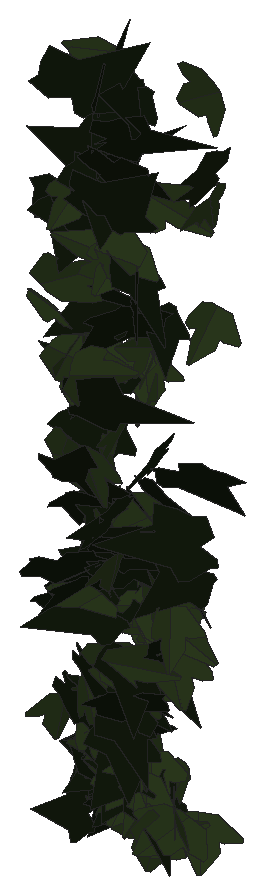
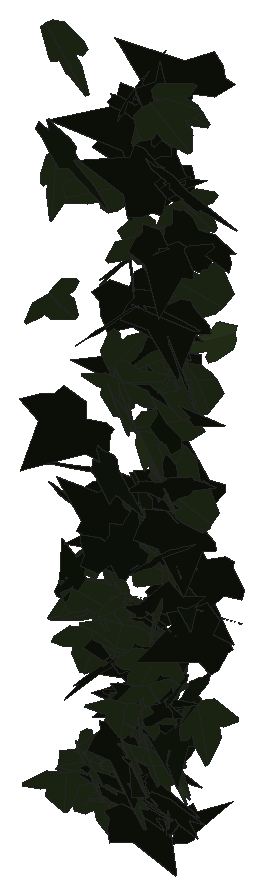
# SketchUp Ruby script. Lengths in inches.
U = 1.inch
M = Sketchup.active_model
def pt(a) = Geom::Point3d.new(a.map { |v| v * U })
def face(e, loops, mat)
  f = e.add_face(loops[0].map { |a| pt(a) })
  loops[1..].each { |l| e.add_face(l.map { |a| pt(a) }).erase! }
  f.material = f.back_material = mat if mat
  f
end
# faces: each face lists its corners as indices into pts; further lists are holes
def faces(e, pts, list, mat = nil) = list.each { |f| face(e, (f[0].is_a?(Array) ? f : [f]).map { |l| l.map { |i| pts[i] } }, mat) }
# xy, xz, yz: faces in a plane at the given z, y or x. An outline is a flat list of corners, or four numbers for a rectangle; further outlines are holes
def ring(l) = l.size == 4 ? [[l[0], l[1]], [l[2], l[1]], [l[2], l[3]], [l[0], l[3]]] : l.each_slice(2).to_a
def flat(e, list, mat, &to3) = list.each { |f| face(e, (f[0].is_a?(Array) ? f : [f]).map { |l| ring(l).map { |u, v| to3.(u, v) } }, mat) }
def xy(e, z, list, mat = nil) = flat(e, list, mat) { |x, y| [x, y, z] }
def xz(e, y, list, mat = nil) = flat(e, list, mat) { |x, z| [x, y, z] }
def yz(e, x, list, mat = nil) = flat(e, list, mat) { |y, z| [x, y, z] }
def lines(e, pts, list) = list.each { |a, b| e.add_line(pt(pts[a]), pt(pts[b])) }
# prism: a flat outline (further loops are holes) pulled along v
def prism(e, loops, v, mat = nil)
  f = face(e, loops, mat); d = Geom::Vector3d.new(v.map { |x| x * U })
  f.pushpull(f.normal.samedirection?(d) ? d.length : -d.length)
end
def box(e, o, s, mat = nil) = prism(e, [[o, [o[0] + s[0], o[1], o[2]], [o[0] + s[0], o[1] + s[1], o[2]], [o[0], o[1] + s[1], o[2]]]], [0, 0, s[2]], mat)
def at(x, y, z, deg = 0) = Geom::Transformation.translation(pt([x, y, z])) * Geom::Transformation.rotation(ORIGIN, Z_AXIS, deg.degrees)
def axes(o, x, y, z) = Geom::Transformation.new([*x, 0, *y, 0, *z, 0, *pt(o).to_a, 1])
def part(name) = M.definitions.add(name)
# library, detail: a bought-in or finely detailed component or shape, given as its bounding box
def library(name, o, s) = part(name).tap { |d| box(d.entities, o, s) }
def detail(e, o, s) = box(e.add_group.entities, o, s)
def put(e, d, t, mat = nil) = e.add_instance(d, t).tap { |i| i.material = mat if mat }
def group(e, t, mat = nil) = e.add_group.tap { |g| g.transformation = t; g.material = mat if mat }.entities
root = M.entities
M.materials.add("1026 AP 7946 SUNNY SIDE UP").color = [254, 231, 186]
M.materials.add("efeu1").color = [18, 25, 13]
M.materials.add("efeu2").color = [43, 57, 29]
c1 = part("ivyleaf_10")
p = [[0,0.5,-0.03],[-0.0625,2.02,-0.43],[-0.19,2.01,-0.46],[-0.54,1.05,-0.29],[-0.52,0.625,-0.18],[-0.83,0.76,-0.28],
  [-1.16,0.64,-0.33],[-1.15,0.33,-0.24],[-0.77,-0.39,0.02],[-0.3,-0.51,0.16],[0.04,-0.48,0.23],[-0.02,2.01,-0.4375],
  [-0.06,2.01,-0.43],[0.04,-0.49,0.23],[0.67,-0.49,0.14],[1.38,0.36,-0.2],[1.375,0.51,-0.24],[0.81,0.65,-0.19],
  [0.62,0.59,-0.15],[0.6,1.09,-0.28],[0.5,1.23,-0.31]]
faces(c1.entities,p,[[0,1,2,3,4,5,6,7,8,9,10],[11,12,0,13,14,15,16,17,18,19,20]],"efeu2")
c2 = part("ivyleaf_9")
p = [[1.54,2.16,1.25],[1.36,2.04,1.19],[-0.21,0.99,0.68],[-0.71,1.11,0.82],[-0.85,0.86,0.67],[-0.8,0.17,0.21],
  [-0.9,-0.01,0.1],[-0.67,-0.16,-0.02],[-0.08,-0.08,-0.05],[-0.03,-0.6,-0.4],[0.65,-0.88,-0.66],[0.83,-0.6,-0.49],
  [1.29,-0.42,-0.43],[1.8125,-0.07,-0.26],[1.21,0.44,0.15]]
faces(c2.entities,p,[[0,1,2,3,4,5,6,7,8,9,10,11,12,13,14]],"efeu1")
put(root,c1,axes([144.89,211.45,272.21],[-0.0227,-0.33557,-0.0993],[-0.00987,0.0948,-0.34531],[0.54808,-0.01219,-0.01033]),"1026 AP 7946 SUNNY SIDE UP")
put(root,c2,axes([144.43,211.41,274.46],[0.30353,0.02891,0.30855],[0.47283,-0.01316,-0.19853],[-0.00717,0.35594,-0.03031]),"1026 AP 7946 SUNNY SIDE UP")
put(root,c2,axes([146.07,211.7,272.7],[-0.47124,0.04372,0.17685],[-0.27106,-0.14791,-0.27249],[0.06248,-0.31197,0.15171]),"1026 AP 7946 SUNNY SIDE UP")
put(root,c1,axes([145.74,211.61,271.51],[0.1198,0.3075,-0.11357],[-0.01937,-0.11221,-0.32669],[-0.51421,0.07587,-0.01416]),"1026 AP 7946 SUNNY SIDE UP")
put(root,c2,axes([144.91,211.76,270.46],[-0.00995,-0.3277,0.08389],[-0.01626,-0.08308,-0.33803],[0.53141,-0.00868,-0.00877]),"1026 AP 7946 SUNNY SIDE UP")
put(root,c2,axes([145.07,211.5,270.11],[0.11535,0.2613,-0.1527],[-0.10067,-0.13703,-0.27952],[-0.4627,0.09496,0.02275]),"1026 AP 7946 SUNNY SIDE UP")
put(root,c2,axes([144.54,211.72,271.16],[-0.46229,-0.00111,0.10729],[-0.1491,-0.12621,-0.27787],[0.06777,-0.28523,0.12054]),"1026 AP 7946 SUNNY SIDE UP")
put(root,c2,axes([144.67,211.55,277.37],[-0.23254,-0.0056,0.30618],[0.43283,-0.12798,0.13786],[0.17658,0.30634,0.0653]),"1026 AP 7946 SUNNY SIDE UP")
put(root,c1,axes([144.78,211.72,276.63],[0.13157,0.14452,0.3287],[-0.29516,-0.25746,0.16978],[0.4636,-0.20493,0.01482]),"1026 AP 7946 SUNNY SIDE UP")
put(root,c1,axes([144.3,211.65,271.27],[0.37111,0.04813,-0.2058],[-0.30199,-0.05766,-0.24807],[-0.11606,0.30396,-0.01258]),"1026 AP 7946 SUNNY SIDE UP")
put(root,c2,axes([144.24,211.68,271.48],[-0.10547,0.19541,-0.2437],[0.01062,-0.24226,-0.20858],[-0.48369,-0.04793,0.04856]),"1026 AP 7946 SUNNY SIDE UP")
put(root,c1,axes([145.05,211.67,268.77],[0.42892,0.15208,-0.10867],[-0.12973,-0.06997,-0.3215],[-0.26138,0.2843,-0.01876]),"1026 AP 7946 SUNNY SIDE UP")
put(root,c1,axes([144.39,211.37,274.9],[-0.06581,-0.08562,-0.35998],[0.30441,0.29057,-0.09567],[0.47593,-0.19769,0.01141]),"1026 AP 7946 SUNNY SIDE UP")
put(root,c2,axes([144.89,211.82,268.94],[-0.30198,-0.20928,0.09031],[-0.03058,-0.10077,-0.28839],[0.3562,-0.18608,0.05181]),"1026 AP 7946 SUNNY SIDE UP")
put(root,c2,axes([143.98,211.61,269.83],[0.32583,-0.23941,-0.09246],[-0.08205,0.07171,-0.32569],[0.39281,0.21357,0.00867]),"1026 AP 7946 SUNNY SIDE UP")
put(root,c1,axes([143.86,211.64,269.62],[-0.14906,-0.31476,-0.00412],[0.02273,-0.00204,-0.33833],[0.49441,-0.0948,0.01431]),"1026 AP 7946 SUNNY SIDE UP")
put(root,c2,axes([144.93,211.82,276.3125],[-0.03483,-0.05751,-0.32695],[0.45525,-0.14301,0.00505],[-0.22234,-0.28381,0.06156]),"1026 AP 7946 SUNNY SIDE UP")
put(root,c2,axes([143.96,211.45,271.84],[0.32103,0.27951,-0.03092],[-0.00381,-0.0373,-0.35621],[-0.44228,0.2032,-0.01937]),"1026 AP 7946 SUNNY SIDE UP")
put(root,c1,axes([144.05,211.74,277.45],[0.23115,0.20832,-0.19197],[-0.16692,-0.1546,-0.26356],[-0.4079,0.18131,-0.00094]),"1026 AP 7946 SUNNY SIDE UP")
put(root,c2,axes([144.76,211.52,272.72],[-0.22638,0.31416,0.00975],[-0.01086,0.00529,-0.35596],[-0.49401,-0.14408,0.00335]),"1026 AP 7946 SUNNY SIDE UP")
put(root,c2,axes([144.18,211.48,279.05],[-0.16959,-0.00997,0.37282],[0.55756,0.07355,0.11137],[-0.11526,0.37045,-0.00982]),"1026 AP 7946 SUNNY SIDE UP")
put(root,c2,axes([144.82,211.78,269.35],[-0.09803,-0.29363,-0.01702],[0.01486,0.01318,-0.30909],[0.46206,-0.06272,0.00633]),"1026 AP 7946 SUNNY SIDE UP")
put(root,c1,axes([144.27,211.64,273.47],[-0.46605,0.12286,-0.0671],[0.07628,-0.0541,-0.32933],[-0.20547,-0.29876,0.02994]),"1026 AP 7946 SUNNY SIDE UP")
put(root,c1,axes([145.75,211.72,268.33],[0.41979,0.05405,-0.17891],[-0.26358,-0.04797,-0.28064],[-0.11216,0.31502,-0.0101]),"1026 AP 7946 SUNNY SIDE UP")
put(root,c1,axes([145.15,211.875,268.51],[-0.09521,-0.19556,0.2531],[0.08334,-0.25406,-0.19548],[0.48806,0.00523,0.08276]),"1026 AP 7946 SUNNY SIDE UP")
put(root,c2,axes([144.98,211.73,275.8125],[-0.04606,0.23487,-0.27374],[-0.03539,-0.26864,-0.24243],[-0.55809,-0.00235,0.03797]),"1026 AP 7946 SUNNY SIDE UP")
put(root,c1,axes([143.45,211.65,275.56],[0.17156,-0.25707,0.06013],[0.39377,0.08037,-0.11424],[0.13112,0.095,0.2644]),"1026 AP 7946 SUNNY SIDE UP")
put(root,c2,axes([146,211.77,272.26],[-0.50513,0.05209,-0.0651],[0.08997,-0.04192,-0.33393],[-0.09263,-0.32477,0.03068]),"1026 AP 7946 SUNNY SIDE UP")
put(root,c2,axes([144.02,211.76,272.95],[0.47426,-0.03134,0.08136],[-0.11757,0.04179,0.31081],[-0.064,-0.30902,0.03193]),"1026 AP 7946 SUNNY SIDE UP")
put(root,c2,axes([144.0625,211.88,267.84],[-0.09074,-0.04802,0.27688],[-0.28488,-0.19915,-0.07782],[0.32173,-0.18988,0.00919]),"1026 AP 7946 SUNNY SIDE UP")
put(root,c1,axes([143.83,211.57,276.02],[-0.20719,-0.15622,0.28667],[0.2926,0.20814,0.2117],[-0.40914,0.22796,0.00623]),"1026 AP 7946 SUNNY SIDE UP")
put(root,c1,axes([144.93,211.48,270.57],[0.12643,0.02144,0.32966],[0.23583,0.28896,-0.0571],[-0.44554,0.15903,0.06333]),"1026 AP 7946 SUNNY SIDE UP")
put(root,c2,axes([144.74,211.8,269.59],[0.05581,-0.29831,-0.02866],[0.0217,0.02791,-0.30883],[0.47036,0.03411,0.01765]),"1026 AP 7946 SUNNY SIDE UP")
put(root,c1,axes([144.3,211.63,269.97],[-0.01626,0.33061,0.03827],[-0.06651,0.0337,-0.33793],[-0.51855,-0.01469,0.04215]),"1026 AP 7946 SUNNY SIDE UP")
put(root,c2,axes([144.12,211.8,268.8],[0.22437,-0.26437,0.01526],[-0.00302,-0.01956,-0.3094],[0.41648,0.14228,-0.01047]),"1026 AP 7946 SUNNY SIDE UP")
put(root,c1,axes([144.63,211.79,269.04],[-0.33322,-0.1935,0.13462],[-0.11605,-0.11345,-0.29458],[0.34934,-0.22226,0.03054]),"1026 AP 7946 SUNNY SIDE UP")
put(root,c1,axes([144.37,211.69,269.4],[0.12774,0.31799,0.00764],[0.02219,0.00218,-0.33782],[-0.49959,0.0814,-0.01305]),"1026 AP 7946 SUNNY SIDE UP")
put(root,c1,axes([144.75,211.84,276.69],[0.29609,0.20892,-0.18212],[-0.16955,-0.14216,-0.29029],[-0.39684,0.21662,-0.01186]),"1026 AP 7946 SUNNY SIDE UP")
put(root,c2,axes([144.93,211.88,268.86],[-0.36004,-0.186,-0.01276],[0.03148,-0.0067,-0.30339],[0.29131,-0.22916,0.01701]),"1026 AP 7946 SUNNY SIDE UP")
put(root,c2,axes([144.98,211.54,272.49],[0.35809,0.25794,0.00745],[0.00483,0.00498,-0.35445],[-0.40566,0.22775,0.00236]),"1026 AP 7946 SUNNY SIDE UP")
put(root,c2,axes([144.36,211.92,277.65],[-0.14218,-0.31337,0.01146],[0.00785,-0.01487,-0.33596],[0.49309,-0.09012,0.00865]),"1026 AP 7946 SUNNY SIDE UP")
put(root,c2,axes([144.33,211.59,271.79],[0.02555,0.31294,0.0444],[-0.06607,0.04315,-0.31939],[-0.49191,0.01046,0.0452]),"1026 AP 7946 SUNNY SIDE UP")
put(root,c2,axes([144.72,211.68,278.07],[0.47008,0.0842,-0.16184],[-0.22483,-0.07141,-0.31919],[-0.16843,0.33031,-0.0256]),"1026 AP 7946 SUNNY SIDE UP")
put(root,c2,axes([144.11,211.77,270.22],[0.35858,-0.2191,-0.0963],[-0.11718,0.05548,-0.32526],[0.35495,0.23965,-0.01009]),"1026 AP 7946 SUNNY SIDE UP")
put(root,c1,axes([145.79,211.67,268.52],[-0.26324,0.22159,0.17373],[-0.2213,0.10078,-0.28188],[-0.37642,-0.21421,0.04422]),"1026 AP 7946 SUNNY SIDE UP")
put(root,c1,axes([145.39,211.625,268.03],[-0.11476,-0.0981,0.29304],[0.18706,0.26006,0.12512],[-0.43547,0.13757,-0.02347]),"1026 AP 7946 SUNNY SIDE UP")
put(root,c2,axes([144.82,211.92,276.47],[0.15948,-0.33075,-0.01898],[-0.02377,0.01266,-0.35615],[0.52018,0.10198,-0.01045]),"1026 AP 7946 SUNNY SIDE UP")
put(root,c2,axes([145.07,211.97,268.34],[0.08236,-0.31394,0.04622],[0.00462,-0.04679,-0.32812],[0.49903,0.05225,-0.00459]),"1026 AP 7946 SUNNY SIDE UP")
put(root,c2,axes([144.83,212.04,278.83],[-0.11578,0.00468,0.32394],[-0.19857,-0.29618,-0.02766],[0.45282,-0.12868,0.07069]),"1026 AP 7946 SUNNY SIDE UP")
put(root,c2,axes([143.7,211.9,277.25],[-0.19955,-0.1001,-0.29884],[0.43708,0.09405,-0.15848],[0.2024,-0.30179,0.0476]),"1026 AP 7946 SUNNY SIDE UP")
put(root,c2,axes([143.87,211.99,276.92],[-0.27109,-0.2359,-0.0123],[0.02941,-0.00056,-0.30059],[0.37014,-0.17273,0.01488]),"1026 AP 7946 SUNNY SIDE UP")
put(root,c1,axes([143.78,211.77,274.84],[-0.19256,-0.06791,-0.29227],[0.44068,0.05652,-0.13843],[0.12518,-0.30344,0.0377]),"1026 AP 7946 SUNNY SIDE UP")
put(root,c2,axes([144.72,211.98,268.86],[-0.43954,-0.0734,0.06198],[-0.08317,-0.03645,-0.29713],[0.12441,-0.28369,0.02034]),"1026 AP 7946 SUNNY SIDE UP")
put(root,c1,axes([145.31,211.86,267.97],[-0.42018,-0.14686,0.06338],[-0.06565,-0.05304,-0.31331],[0.24213,-0.26923,0.02504]),"1026 AP 7946 SUNNY SIDE UP")
put(root,c2,axes([144.44,211.96,275.74],[-0.47524,-0.01458,0.02859],[-0.04087,-0.03536,-0.30996],[0.02777,-0.30145,0.03318]),"1026 AP 7946 SUNNY SIDE UP")
put(root,c1,axes([144.98,211.84,268.9375],[-0.20625,0.26545,-0.02318],[-0.00332,-0.02779,-0.30484],[-0.41908,-0.13042,0.01382]),"1026 AP 7946 SUNNY SIDE UP")
put(root,c2,axes([144.83,211.92,271.72],[0.26227,0.09112,0.25889],[-0.40756,-0.0149,0.18308],[0.09963,-0.30082,0.06742]),"1026 AP 7946 SUNNY SIDE UP")
put(root,c1,axes([144.54,211.92,268.92],[0.44165,0.09446,-0.01587],[-0.00919,-0.0324,-0.30402],[-0.15035,0.27945,-0.02804]),"1026 AP 7946 SUNNY SIDE UP")
put(root,c2,axes([144.83,211.84,270.39],[0.33564,0.22543,0.03474],[-0.06236,-0.00699,0.31885],[0.35265,-0.2158,0.02332]),"1026 AP 7946 SUNNY SIDE UP")
put(root,c1,axes([145.17,211.91,268.96],[0.20195,0.28357,-0.06245],[-0.00767,-0.06593,-0.32026],[-0.45643,0.12657,-0.02225]),"1026 AP 7946 SUNNY SIDE UP")
put(root,c2,axes([144.56,211.69,272.21],[0.08232,0.06124,-0.3348],[0.1751,0.30693,0.07978],[0.49021,-0.11992,0.02773]),"1026 AP 7946 SUNNY SIDE UP")
put(root,c1,axes([144.09,211.91,275.03],[-0.09221,0.29202,-0.06205],[0.00687,-0.06223,-0.3071],[-0.46932,-0.05828,0.0077]),"1026 AP 7946 SUNNY SIDE UP")
put(root,c1,axes([143.76,211.9375,274.59],[-0.04606,-0.31007,0.00879],[0.01913,0.00918,0.3207],[-0.48744,0.02966,0.01176]),"1026 AP 7946 SUNNY SIDE UP")
put(root,c2,axes([144.46,211.73,269.42],[0.02539,0.32457,0.05012],[-0.07478,0.04869,-0.33061],[-0.51019,0.00902,0.05095]),"1026 AP 7946 SUNNY SIDE UP")
put(root,c2,axes([144.6,211.75,278.39],[0.31071,0.03967,0.30087],[0.44369,0.07515,-0.20692],[-0.13262,0.34433,0.01263]),"1026 AP 7946 SUNNY SIDE UP")
put(root,c2,axes([144.02,211.92,274.05],[0.11652,0.25885,0.14764],[-0.09576,-0.12969,0.27584],[0.45414,-0.09376,0.02028]),"1026 AP 7946 SUNNY SIDE UP")
put(root,c1,axes([144.17,212.12,279.17],[-0.1529,-0.13432,0.26367],[-0.16273,-0.23681,-0.16942],[0.4255,-0.13883,0.02995]),"1026 AP 7946 SUNNY SIDE UP")
put(root,c1,axes([143.95,212.1,268.92],[0.20431,-0.22978,0.16112],[0.10531,-0.14316,-0.27257],[0.42538,0.14581,-0.00991]),"1026 AP 7946 SUNNY SIDE UP")
put(root,c1,axes([144.5,212.04,273.79],[0.062,-0.29019,0.05488],[0.00081,-0.05534,-0.30194],[0.46439,0.03884,-0.0068]),"1026 AP 7946 SUNNY SIDE UP")
put(root,c2,axes([144.21,211.9,275.88],[0.32307,0.13237,-0.19886],[-0.25092,-0.11005,-0.25239],[-0.27057,0.26011,-0.00339]),"1026 AP 7946 SUNNY SIDE UP")
put(root,c2,axes([144.91,212.05,269.67],[-0.23811,-0.16435,-0.16914],[-0.19235,-0.10889,0.2292],[-0.30932,0.19423,-0.01232]),"1026 AP 7946 SUNNY SIDE UP")
put(root,c1,axes([144.28,211.85,268.51],[-0.1739,0.17838,0.19408],[-0.22141,0.12945,-0.21181],[-0.34126,-0.17489,0.03852]),"1026 AP 7946 SUNNY SIDE UP")
put(root,c1,axes([144.56,211.88,269.27],[0.17735,0.2207,0.16635],[0.12773,0.13833,-0.25439],[-0.40937,0.13877,-0.0073]),"1026 AP 7946 SUNNY SIDE UP")
put(root,c1,axes([144.73,212,268.86],[-0.42648,0.10548,0.05362],[-0.11532,-0.05118,-0.29047],[-0.14406,-0.27128,0.07376]),"1026 AP 7946 SUNNY SIDE UP")
put(root,c2,axes([144.55,212.14,278.95],[-0.45222,-0.09368,-0.09777],[0.15184,0.00745,-0.31075],[0.14375,-0.30259,0.02067]),"1026 AP 7946 SUNNY SIDE UP")
put(root,c1,axes([144.4,211.99,270.38],[-0.37831,-0.12046,-0.1001],[0.15224,0.02135,-0.27607],[0.18899,-0.25834,0.02201]),"1026 AP 7946 SUNNY SIDE UP")
put(root,c1,axes([144.56,212.03,267.79],[-0.45491,-0.02423,0.08048],[0.11801,0.03678,0.29777],[-0.05165,0.29744,-0.02848]),"1026 AP 7946 SUNNY SIDE UP")
put(root,c1,axes([144.25,212.03,272.17],[-0.40866,0.18256,0.03955],[-0.14741,-0.0727,-0.30637],[-0.25322,-0.2523,0.11452]),"1026 AP 7946 SUNNY SIDE UP")
put(root,c1,axes([143.54,212.05,273.01],[-0.18459,0.00857,0.30537],[0.46592,0.01457,0.12057],[-0.01635,0.31844,-0.01187]),"1026 AP 7946 SUNNY SIDE UP")
put(root,c2,axes([145.71,211.88,273.61],[0.47454,0.15109,0.03882],[0.06461,0.00006,-0.34719],[-0.23584,0.30403,-0.017]),"1026 AP 7946 SUNNY SIDE UP")
put(root,c2,axes([144.5,212.25,268.68],[-0.03475,-0.06692,0.27557],[0.04252,-0.26796,-0.06824],[0.43206,0.02099,0.02888]),"1026 AP 7946 SUNNY SIDE UP")
put(root,c2,axes([144.6,212.11,271.22],[-0.40995,0.1074,0.0417],[-0.07587,-0.01306,-0.28889],[-0.16338,-0.26342,0.02952]),"1026 AP 7946 SUNNY SIDE UP")
put(root,c2,axes([144.13,211.98,277.86],[-0.24204,0.17001,0.22365],[-0.26871,0.13491,-0.23392],[-0.33875,-0.22849,0.02575]),"1026 AP 7946 SUNNY SIDE UP")
put(root,c2,axes([144.37,212.02,274.36],[-0.12622,0.11455,0.27622],[-0.38496,0.12336,-0.12939],[-0.24725,-0.25054,0.06046]),"1026 AP 7946 SUNNY SIDE UP")
put(root,c2,axes([143.54,211.86,271.05],[0.29152,0.17043,0.20174],[0.25883,0.10738,-0.25747],[-0.31418,0.2466,-0.02491]),"1026 AP 7946 SUNNY SIDE UP")
put(root,c1,axes([144.82,212.3,275.04],[-0.05562,-0.08484,-0.29346],[-0.16163,-0.26516,0.09312],[-0.43774,0.10869,0.00291]),"1026 AP 7946 SUNNY SIDE UP")
put(root,c1,axes([144.52,211.99,268.33],[0.15992,0.09378,0.27937],[0.35394,0.15145,-0.14032],[-0.27854,0.24629,-0.0179]),"1026 AP 7946 SUNNY SIDE UP")
put(root,c1,axes([143.9,212.02,274.32],[0.2165,0.1042,0.25699],[0.34388,0.12051,-0.17592],[-0.24843,0.25762,-0.01956]),"1026 AP 7946 SUNNY SIDE UP")
put(root,c2,axes([144.2,212.11,269.9375],[0.32865,-0.07529,0.15376],[0.2001,-0.08433,-0.22726],[0.17138,0.24285,-0.02952]),"1026 AP 7946 SUNNY SIDE UP")
put(root,c1,axes([145.8,212.12,268.16],[0.32798,0.22954,-0.0163],[0.00531,-0.02616,-0.319],[-0.36189,0.20765,-0.01945]),"1026 AP 7946 SUNNY SIDE UP")
put(root,c1,axes([145.29,212.17,270.51],[-0.46568,-0.11547,-0.04769],[0.13999,-0.11523,-0.29554],[0.13608,-0.27661,0.14084]),"1026 AP 7946 SUNNY SIDE UP")
put(root,c2,axes([143.98,212,272.63],[0.1435,0.272,-0.08053],[-0.03817,-0.07594,-0.296],[-0.44404,0.09443,-0.00058]),"1026 AP 7946 SUNNY SIDE UP")
put(root,c1,axes([144.59,212.14,269.74],[-0.46107,-0.02924,0.06984],[-0.09206,-0.07815,-0.29531],[0.07112,-0.29068,0.07053]),"1026 AP 7946 SUNNY SIDE UP")
put(root,c1,axes([145.01,212.13,272.63],[0.38594,-0.0485,-0.20034],[-0.30239,0.02805,-0.25746],[0.08726,0.31172,-0.00612]),"1026 AP 7946 SUNNY SIDE UP")
put(root,c2,axes([144.32,211.88,278.84],[0.03631,-0.07071,0.38943],[0.22141,0.35438,0.06144],[-0.56337,0.13471,0.04924]),"1026 AP 7946 SUNNY SIDE UP")
put(root,c1,axes([144.34,212.1875,272.01],[-0.00367,-0.02253,-0.31026],[0.42717,-0.13144,0.0072],[-0.207,-0.27084,0.02034]),"1026 AP 7946 SUNNY SIDE UP")
put(root,c1,axes([146.03,212.02,279.47],[0.33414,-0.14174,-0.26549],[-0.2694,0.19756,-0.25713],[0.37454,0.26856,0.0519]),"1026 AP 7946 SUNNY SIDE UP")
put(root,c2,axes([145.24,212.19,268.4],[-0.40043,0.06178,0.1317],[-0.20438,0.00239,-0.26867],[-0.08858,-0.28478,0.02457]),"1026 AP 7946 SUNNY SIDE UP")
put(root,c1,axes([144.95,212.3,270.875],[-0.07081,0.00554,0.29243],[-0.26428,-0.23211,-0.02416],[0.35973,-0.16943,0.03981]),"1026 AP 7946 SUNNY SIDE UP")
put(root,c1,axes([144.83,212.33,271.11],[-0.04214,0.06886,0.27426],[-0.06801,-0.26482,0.06462],[0.4264,-0.03543,0.03741]),"1026 AP 7946 SUNNY SIDE UP")
put(root,c2,axes([144.52,212.16,268.07],[0.05497,0.1972,-0.20275],[-0.07354,-0.19252,-0.20725],[-0.43313,0.05771,0.00945]),"1026 AP 7946 SUNNY SIDE UP")
put(root,c1,axes([144.25,212.21,270.12],[0.28729,0.19063,-0.10061],[-0.08647,-0.08378,-0.27194],[-0.32632,0.19004,-0.01652]),"1026 AP 7946 SUNNY SIDE UP")
put(root,c1,axes([144.57,212.19,274.71],[0.1884,0.13406,0.25853],[-0.36565,-0.10937,0.17446],[0.25594,-0.25493,0.05893]),"1026 AP 7946 SUNNY SIDE UP")
put(root,c1,axes([145.09,212.01,271.56],[0.16128,-0.06919,-0.28611],[-0.23657,0.23745,-0.11697],[0.38214,0.1762,0.04834]),"1026 AP 7946 SUNNY SIDE UP")
put(root,c2,axes([143.71,212.33,275.37],[-0.21314,0.00242,-0.28257],[0.39656,-0.11924,-0.13018],[-0.16965,-0.28177,0.05072]),"1026 AP 7946 SUNNY SIDE UP")
put(root,c1,axes([145.1,212.05,277.49],[0.20792,0.08877,0.28674],[0.32027,0.19025,-0.16137],[-0.32828,0.24183,0.02418]),"1026 AP 7946 SUNNY SIDE UP")
put(root,c1,axes([144.36,212.03,273.37],[-0.03257,0.11367,0.28233],[-0.38618,0.1465,-0.08106],[-0.26008,-0.23177,0.085]),"1026 AP 7946 SUNNY SIDE UP")
put(root,c1,axes([145.02,212.18,268.86],[-0.10318,0.2685,0.02964],[0.01636,-0.0255,0.28457],[0.42405,0.06632,-0.00377]),"1026 AP 7946 SUNNY SIDE UP")
put(root,c2,axes([144.3125,212.15,269.88],[-0.03313,-0.08132,-0.26291],[0.26692,0.19337,-0.07693],[0.32488,-0.16716,0.03639]),"1026 AP 7946 SUNNY SIDE UP")
put(root,c1,axes([145.15,212.07,271.2],[0.21424,0.15252,0.2255],[0.21372,0.17069,-0.20952],[-0.35969,0.19227,0.00983]),"1026 AP 7946 SUNNY SIDE UP")
put(root,c1,axes([144.59,212.07,269.8],[0.12979,-0.17193,-0.21749],[-0.07701,0.20661,-0.19275],[0.41992,0.09103,0.03187]),"1026 AP 7946 SUNNY SIDE UP")
put(root,c2,axes([144.09,212.41,272.24],[-0.17483,-0.23984,0.11975],[-0.05722,-0.11259,-0.27266],[0.4161,-0.11625,0.01282]),"1026 AP 7946 SUNNY SIDE UP")
put(root,c2,axes([144.07,212.13,276.95],[0.38969,-0.01325,-0.20978],[-0.32023,-0.03433,-0.25334],[-0.01828,0.31887,-0.0341]),"1026 AP 7946 SUNNY SIDE UP")
put(root,c1,axes([145.19,212.12,271.05],[0.2381,0.14047,0.25785],[0.34068,0.12829,-0.20913],[-0.29432,0.26214,-0.03348]),"1026 AP 7946 SUNNY SIDE UP")
put(root,c1,axes([144.22,212.21,268.95],[-0.21777,-0.02846,-0.26678],[0.40844,-0.03514,-0.13943],[-0.02798,-0.29142,0.04112]),"1026 AP 7946 SUNNY SIDE UP")
put(root,c2,axes([144.69,212.33,268.35],[-0.45316,-0.03239,-0.03935],[0.06331,-0.01892,-0.29792],[0.04647,-0.29007,0.0221]),"1026 AP 7946 SUNNY SIDE UP")
put(root,c1,axes([145.36,212.27,268.7],[0.27185,-0.22649,-0.0266],[-0.04707,0.00795,-0.29285],[0.35511,0.17444,-0.01845]),"1026 AP 7946 SUNNY SIDE UP")
put(root,c2,axes([144.89,212.41,275.59],[-0.00908,-0.30006,0.0586],[-0.00302,-0.05856,-0.30952],[0.48071,-0.00604,-0.00084]),"1026 AP 7946 SUNNY SIDE UP")
put(root,c2,axes([144.1,212.36,268.58],[-0.46108,-0.04856,-0.07723],[0.1246,-0.02474,-0.30406],[0.06402,-0.30158,0.03556]),"1026 AP 7946 SUNNY SIDE UP")
put(root,c2,axes([143.9,212.4,273.5],[-0.26999,-0.2403,-0.0204],[0.04101,0.00398,-0.30361],[0.37674,-0.17264,0.01843]),"1026 AP 7946 SUNNY SIDE UP")
put(root,c1,axes([144.12,212.17,271.52],[-0.18328,0.25519,0.07864],[-0.06514,0.06335,-0.28843],[-0.41308,-0.12322,0.01059]),"1026 AP 7946 SUNNY SIDE UP")
put(root,c2,axes([145.42,212.47,271.43],[0.01279,-0.11295,0.26913],[0.0669,-0.25858,-0.11777],[0.44343,0.04227,0.01]),"1026 AP 7946 SUNNY SIDE UP")
put(root,c2,axes([145.92,212.25,278.09],[-0.34612,0.25852,-0.05352],[0.03481,-0.05123,-0.3497],[-0.41363,-0.22064,0.01536]),"1026 AP 7946 SUNNY SIDE UP")
put(root,c1,axes([144.7,212.38,274.45],[0.32852,-0.18553,0.0943],[0.09198,-0.07336,-0.28785],[0.3128,0.21643,-0.01439]),"1026 AP 7946 SUNNY SIDE UP")
put(root,c2,axes([144.51,212.06,268.68],[0.05812,0.13763,0.24578],[0.01969,0.23884,-0.14302],[-0.43157,0.02943,0.02658]),"1026 AP 7946 SUNNY SIDE UP")
put(root,c2,axes([144.63,212.28,268.77],[-0.13141,-0.0542,-0.28387],[-0.40963,-0.09155,0.09952],[-0.16364,0.2727,-0.02117]),"1026 AP 7946 SUNNY SIDE UP")
put(root,c1,axes([144.71,212.29,270.91],[0.3814,0.13765,0.04404],[0.07099,0.00532,-0.28672],[-0.21486,0.24611,-0.01654]),"1026 AP 7946 SUNNY SIDE UP")
put(root,c2,axes([144.65,212.16,269.17],[0.1265,0.28372,-0.04272],[-0.01698,-0.04171,-0.30405],[-0.45091,0.08116,-0.00053]),"1026 AP 7946 SUNNY SIDE UP")
put(root,c1,axes([144.27,212.06,278.98],[0.05733,0.10361,0.30491],[-0.12823,0.29026,-0.09282],[-0.47522,-0.06582,0.06183]),"1026 AP 7946 SUNNY SIDE UP")
put(root,c2,axes([144.37,212.08,277.82],[0.06997,0.28183,-0.15045],[-0.04,0.15176,0.29141],[0.49868,-0.02737,0.04449]),"1026 AP 7946 SUNNY SIDE UP")
put(root,c2,axes([144.12,212.23,271.4],[-0.33807,-0.12457,0.15474],[0.18028,0.10151,0.25518],[-0.24936,0.24227,-0.02531]),"1026 AP 7946 SUNNY SIDE UP")
put(root,c2,axes([145.01,212.32,270.24],[0.14148,-0.23775,-0.12185],[-0.03655,0.11593,-0.26058],[0.41499,0.09126,0.01859]),"1026 AP 7946 SUNNY SIDE UP")
put(root,c1,axes([143.96,212.43,279.18],[-0.27615,-0.18216,0.16909],[-0.11358,-0.15579,-0.25704],[0.36958,-0.18399,0.04734]),"1026 AP 7946 SUNNY SIDE UP")
put(root,c1,axes([145.26,212.4,271.33],[0.27431,0.05789,-0.21985],[-0.31895,-0.06738,-0.18975],[-0.13968,0.26754,0.00152]),"1026 AP 7946 SUNNY SIDE UP")
put(root,c1,axes([145.77,212.46,275.75],[0.17016,0.23398,-0.21102],[-0.1194,-0.19188,-0.26654],[-0.47559,0.13189,-0.00858]),"1026 AP 7946 SUNNY SIDE UP")
put(root,c1,axes([144.56,212.33,269.12],[0.22744,-0.23721,-0.08247],[-0.08541,0.05892,-0.28545],[0.38358,0.15377,-0.01466]),"1026 AP 7946 SUNNY SIDE UP")
put(root,c2,axes([144.83,212.46,272.625],[0.10755,-0.11373,0.25296],[0.25768,-0.18497,-0.13601],[0.33976,0.17628,0.02308]),"1026 AP 7946 SUNNY SIDE UP")
put(root,c1,axes([144.63,212.37,274.71],[0.4332,0.07236,0.06888],[0.11072,-0.00746,-0.29241],[-0.10773,0.28331,-0.02352]),"1026 AP 7946 SUNNY SIDE UP")
put(root,c1,axes([144.58,212.36,269.77],[0.36351,0.14942,0.02644],[0.05073,-0.00433,-0.28277],[-0.2327,0.23247,-0.02034]),"1026 AP 7946 SUNNY SIDE UP")
put(root,c1,axes([145.84,212.26,277.64],[-0.06528,-0.29752,-0.16098],[0.02403,0.15392,-0.30852],[0.52664,-0.0439,-0.00588]),"1026 AP 7946 SUNNY SIDE UP")
put(root,c2,axes([144.93,212.42,273.43],[-0.2699,0.16403,-0.16453],[0.15027,-0.13133,-0.24411],[-0.32825,-0.19499,0.02353]),"1026 AP 7946 SUNNY SIDE UP")
put(root,c1,axes([144.41,212.23,269.26],[-0.13517,0.13306,0.23299],[-0.32625,0.10999,-0.14777],[-0.2509,-0.2147,0.06662]),"1026 AP 7946 SUNNY SIDE UP")
put(root,c1,axes([144.59,212.38,268.59],[0.32522,-0.1844,-0.05932],[-0.0853,0.02392,-0.28472],[0.29102,0.21308,-0.01717]),"1026 AP 7946 SUNNY SIDE UP")
put(root,c1,axes([144.7,212.36,274.8],[0.21933,-0.2489,-0.07358],[-0.06036,0.05873,-0.29355],[0.40205,0.1446,-0.00393]),"1026 AP 7946 SUNNY SIDE UP")
put(root,c2,axes([144.71,212.5,272.06],[0.40365,-0.25002,0.08023],[-0.05829,0.07526,0.36853],[-0.4083,-0.25792,0.02671]),"1026 AP 7946 SUNNY SIDE UP")
